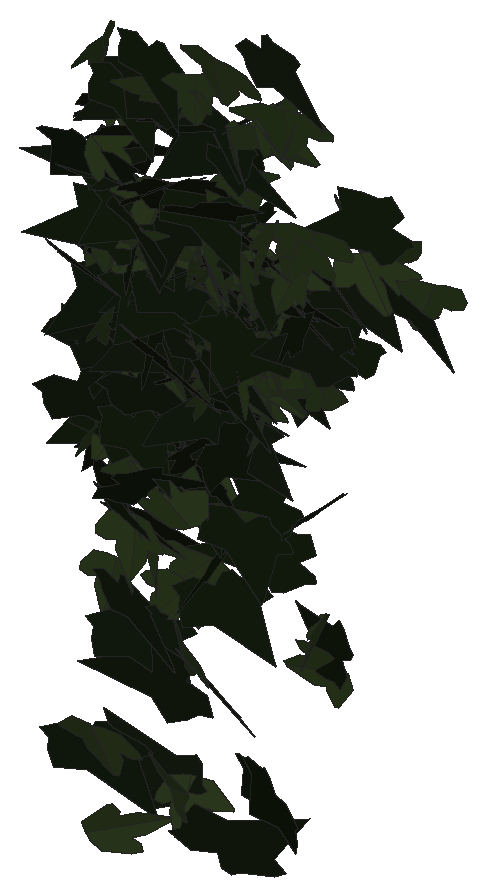
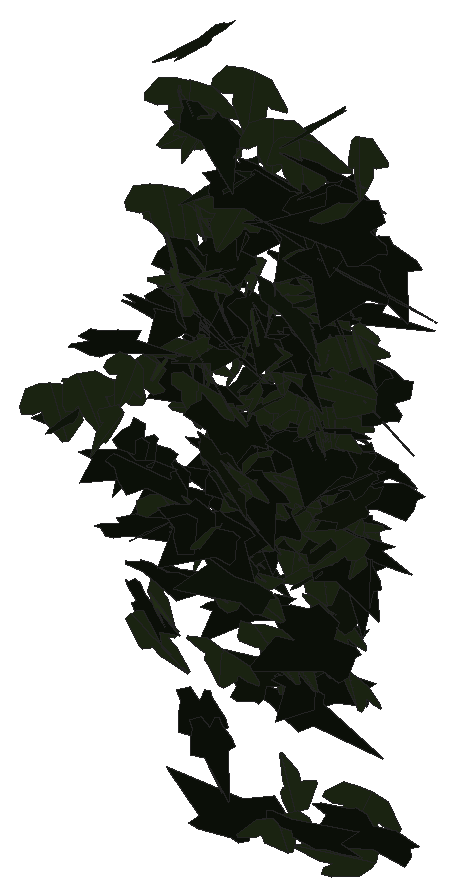
# SketchUp Ruby script. Lengths in millimetres.
U = 1.mm
M = Sketchup.active_model
def pt(a) = Geom::Point3d.new(a.map { |v| v * U })
def face(e, loops, mat)
  f = e.add_face(loops[0].map { |a| pt(a) })
  loops[1..].each { |l| e.add_face(l.map { |a| pt(a) }).erase! }
  f.material = f.back_material = mat if mat
  f
end
# faces: each face lists its corners as indices into pts; further lists are holes
def faces(e, pts, list, mat = nil) = list.each { |f| face(e, (f[0].is_a?(Array) ? f : [f]).map { |l| l.map { |i| pts[i] } }, mat) }
# xy, xz, yz: faces in a plane at the given z, y or x. An outline is a flat list of corners, or four numbers for a rectangle; further outlines are holes
def ring(l) = l.size == 4 ? [[l[0], l[1]], [l[2], l[1]], [l[2], l[3]], [l[0], l[3]]] : l.each_slice(2).to_a
def flat(e, list, mat, &to3) = list.each { |f| face(e, (f[0].is_a?(Array) ? f : [f]).map { |l| ring(l).map { |u, v| to3.(u, v) } }, mat) }
def xy(e, z, list, mat = nil) = flat(e, list, mat) { |x, y| [x, y, z] }
def xz(e, y, list, mat = nil) = flat(e, list, mat) { |x, z| [x, y, z] }
def yz(e, x, list, mat = nil) = flat(e, list, mat) { |y, z| [x, y, z] }
def lines(e, pts, list) = list.each { |a, b| e.add_line(pt(pts[a]), pt(pts[b])) }
# prism: a flat outline (further loops are holes) pulled along v
def prism(e, loops, v, mat = nil)
  f = face(e, loops, mat); d = Geom::Vector3d.new(v.map { |x| x * U })
  f.pushpull(f.normal.samedirection?(d) ? d.length : -d.length)
end
def box(e, o, s, mat = nil) = prism(e, [[o, [o[0] + s[0], o[1], o[2]], [o[0] + s[0], o[1] + s[1], o[2]], [o[0], o[1] + s[1], o[2]]]], [0, 0, s[2]], mat)
def at(x, y, z, deg = 0) = Geom::Transformation.translation(pt([x, y, z])) * Geom::Transformation.rotation(ORIGIN, Z_AXIS, deg.degrees)
def axes(o, x, y, z) = Geom::Transformation.new([*x, 0, *y, 0, *z, 0, *pt(o).to_a, 1])
def part(name) = M.definitions.add(name)
# library, detail: a bought-in or finely detailed component or shape, given as its bounding box
def library(name, o, s) = part(name).tap { |d| box(d.entities, o, s) }
def detail(e, o, s) = box(e.add_group.entities, o, s)
def put(e, d, t, mat = nil) = e.add_instance(d, t).tap { |i| i.material = mat if mat }
def group(e, t, mat = nil) = e.add_group.tap { |g| g.transformation = t; g.material = mat if mat }.entities
root = M.entities
M.materials.add("efeu1").color = [18, 25, 13]
M.materials.add("efeu2").color = [43, 57, 29]
c1 = part("ivyleaf_9")
p = [[39.1,54.8,31.7],[34.5,51.8,30.2],[-5.3,25.2,17.3],[-17.9,28.3,20.9],[-21.6,21.7,17],[-20.2,4.3,5.3],
  [-22.9,-0.3,2.5],[-17.1,-4,-0.6],[-2,-2.1,-1.2],[-0.7,-15.4,-10.1],[16.6,-22.3,-16.7],[21.1,-15.1,-12.5],
  [32.7,-10.7,-11],[46.1,-1.8,-6.6],[30.8,11.2,3.8]]
faces(c1.entities,p,[[0,1,2,3,4,5,6,7,8,9,10,11,12,13,14]],"efeu1")
c2 = part("ivyleaf_10")
p = [[0,12.8,-0.8],[-1.5,51.3,-10.9],[-4.9,51,-11.6],[-13.6,26.5,-7.3],[-13.2,15.9,-4.6],[-21.1,19.3,-7.2],
  [-29.5,16.3,-8.3],[-29.2,8.3,-6.2],[-19.7,-9.8,0.5],[-7.6,-13,4],[1,-12.2,5.8],[-0.4,51.1,-11.1],
  [-1.5,51.1,-10.9],[1,-12.4,5.9],[16.9,-12.4,3.5],[35.1,9.1,-5.1],[35,12.9,-6.1],[20.5,16.4,-4.9],
  [15.8,15,-3.8],[15.3,27.6,-7.1],[12.8,31.3,-7.8]]
faces(c2.entities,p,[[0,1,2,3,4,5,6,7,8,9,10],[11,12,0,13,14,15,16,17,18,19,20]],"efeu2")
put(root,c1,axes([4036.5,844.8,2425.9],[0.72675,0.87653,-0.35288],[-0.34842,-0.30477,-0.95512],[-1.76426,0.42126,0.04326]))
put(root,c1,axes([3981.4,834.6,2057.9],[0.12085,0.58103,-0.82301],[0.24723,0.81303,0.58402],[1.90136,-0.14265,-0.02363]))
put(root,c1,axes([4072.6,839.5,2412.5],[1.22858,0.73783,0.06675],[0.08455,0.04982,-0.98036],[-1.40743,0.64706,-0.00063]))
put(root,c2,axes([3948.9,851.6,2241.1],[0.13677,-0.95686,-0.27886],[0.1005,0.28284,-0.95693],[1.89418,0.05408,0.0709]))
put(root,c2,axes([4040.7,853.5,2035.3],[1.2774,0.03768,0.70919],[-1.3479,-0.03699,0.67224],[0.10044,-0.97574,0.0019]))
put(root,c1,axes([3988.9,868.4,2556.6],[0.22412,-1.0127,0.1095],[0.0018,-0.11012,-1.01945],[1.9386,0.11718,-0.01171]))
put(root,c1,axes([4171.5,844.4,1752],[0.80253,-0.05463,-1.11509],[-2.08064,0.22152,-0.42426],[0.43089,1.1714,0.02823]))
put(root,c1,axes([3976.8,874.3,2352.2],[-0.13475,-0.82447,0.54371],[0.33461,-0.54692,-0.80645],[1.8496,0.03888,0.1855]))
put(root,c2,axes([4017.8,867.2,1695],[-0.99724,0.2867,0.78315],[1.16495,-0.49599,0.59111],[1.07806,0.80118,0.08569]))
put(root,c2,axes([3952.3,841.1,1634.5],[-0.24236,-0.32235,0.95032],[0.62463,0.89188,0.3465],[-1.80484,0.35196,-0.0077]))
put(root,c2,axes([4148.8,866.1,2399.1],[0.28682,-0.92178,0.36124],[0.32407,-0.33582,-0.92796],[1.85616,0.20107,0.1062]))
put(root,c1,axes([3973.5,858.2,2216],[1.68374,-0.52294,0.2093],[0.32287,-0.12423,-1.02749],[1.02224,0.90058,-0.0202]))
put(root,c1,axes([3957.6,871.3,2336.3],[-1.4048,-0.23105,0.65374],[-1.13334,-0.27786,-0.77057],[0.67595,-0.94604,0.06666]))
put(root,c1,axes([3986.4,873.6,2369.2],[-1.49607,-0.49452,0.32912],[-0.39656,-0.28168,-0.92089],[1.05873,-0.8043,0.12015]))
put(root,c1,axes([4084.2,865.5,1993.1],[-0.9583,0.53268,-0.69719],[0.87608,-0.52394,-0.73276],[-1.42157,-0.68197,0.0184]))
put(root,c1,axes([4062.3,865.2,2408.9],[-0.24638,-0.92337,-0.34098],[0.35125,0.31505,-0.92321],[1.84012,-0.18377,0.13057]))
put(root,c1,axes([4003,868.6,2367.5],[-1.35838,-0.18844,-0.70116],[1.35902,-0.00441,-0.7257],[0.24985,-1.00051,0.13525]))
put(root,c2,axes([3996.7,857,2343.4],[-1.81782,-0.12192,-0.11588],[0.22257,-0.00111,-0.96276],[0.23009,-0.96214,0.0158]))
put(root,c1,axes([4145,862.2,2611.8],[0.80477,-0.89334,-0.27629],[-0.06936,0.28725,-0.98456],[1.77832,0.41548,0.08663]))
put(root,c1,axes([3923.6,855.3,2422.1],[0.91515,0.32099,-0.82246],[-1.40893,-0.36372,-0.57477],[-0.91558,0.88054,0.0624]))
put(root,c2,axes([4104.6,868.2,2345.1],[-0.89759,0.60758,-0.59573],[0.43993,-0.56402,-0.75824],[-1.55855,-0.50912,0.12906]))
put(root,c1,axes([3949.2,870.4,1908.8],[0.8109,-0.98165,0.06298],[0.05458,-0.05621,-1.07013],[1.87133,0.42702,0.00392]))
put(root,c1,axes([4054.5,877,1834.2],[0.44139,-0.68251,0.66954],[0.58544,-0.59906,-0.71722],[1.72288,0.37842,0.07218]))
put(root,c1,axes([3968,869.8,2112],[0.0486,-0.93186,-0.28019],[0.05446,0.28089,-0.93156],[1.85115,0.0162,0.03476]))
put(root,c2,axes([4049.6,854.3,1877],[-1.15947,0.60562,0.52098],[-0.74389,0.34544,-0.85863],[-1.32601,-0.72335,0.02614]))
put(root,c2,axes([3937.3,853.8,2431.4],[0.17379,0.88481,0.46957],[0.02273,0.47053,-0.88892],[-1.90628,0.08628,0.03221]))
put(root,c2,axes([3987.7,870.1,2336.3],[1.55558,0.37506,-0.39642],[-0.705,-0.14296,-0.89901],[-0.7627,0.89709,0.02247]))
put(root,c2,axes([3997.5,876.6,2389.3],[-1.02684,-0.76061,0.36563],[0.18223,-0.48633,-0.87041],[1.59579,-0.43389,0.33467]))
put(root,c2,axes([4086.9,861.5,2574.8],[-1.82751,0.28164,0.17703],[-0.30686,0.07902,-1.00023],[-0.55379,-0.97321,-0.02998]))
put(root,c1,axes([3951,875.9,2504.7],[0.02335,-1.00353,-0.14543],[-0.02007,0.14531,-1.00357],[1.92976,0.01365,-0.00868]))
put(root,c1,axes([3993.4,875.7,2510.8],[-1.89727,0.00409,0.06429],[-0.12256,-0.08931,-0.99288],[0.00321,-0.99495,0.08939]))
put(root,c2,axes([4080.3,857.8,2339.1],[-0.8045,0.87477,0.34227],[-0.29796,0.30447,-0.97151],[-1.76276,-0.4507,0.00801]))
put(root,c1,axes([4108.7,877.5,2034.4],[-0.35683,-0.97188,-0.17149],[0.05849,0.16873,-0.9898],[1.87735,-0.18998,-0.00176]))
put(root,c2,axes([4014.2,867.1,2517.6],[-1.74926,-0.38725,0.12108],[-0.20599,-0.05495,-0.99733],[0.74422,-0.92543,0.00855]))
put(root,c1,axes([4003.2,848.1,2402.1],[0.90694,0.74019,0.50477],[0.36079,0.47548,-0.87621],[-1.66651,0.50576,0.08501]))
put(root,c1,axes([4083.3,876.8,2479.3],[-1.91669,0.01537,-0.0447],[0.08402,-0.03504,-1.00662],[-0.03216,-1.00747,0.03433]))
put(root,c2,axes([3921.8,866.1,1728.4],[-1.74339,0.14415,-0.09368],[0.17706,-0.01147,-0.9273],[-0.27515,-0.92074,-0.00312]))
put(root,c1,axes([4030.1,869.3,1827.5],[-0.39088,-0.09178,-1.05774],[-1.864,-0.39954,0.22484],[-0.78008,1.00068,-0.00725]))
put(root,c2,axes([4099.3,868.8,2490.2],[-0.42358,0.96964,-0.12982],[0.01703,-0.13111,-0.99464],[-1.8618,-0.2218,0.02044]))
put(root,c1,axes([3993.4,885.9,2261.5],[-1.25781,-0.65263,0.2339],[-0.19447,-0.22792,-0.92468],[1.30504,-0.66298,0.08765]))
put(root,c2,axes([4167.5,869.9,2538.4],[-1.82818,-0.33509,0.03934],[-0.06118,-0.02726,-1.01724],[0.6392,-0.961,0.01514]))
put(root,c1,axes([3950.7,882.1,2335.9],[-0.8004,0.14549,-0.8766],[1.53067,-0.35005,-0.44395],[-0.71909,-0.90706,0.03072]))
put(root,c1,axes([4114.5,882.3,2254.5],[-1.54837,-0.48363,-0.08834],[0.13424,0.05422,-0.9464],[0.92599,-0.81655,-0.01052]))
put(root,c2,axes([3925.7,866,2549.1],[-0.15213,-0.92921,-0.42172],[0.09813,0.41879,-0.93253],[1.9396,-0.09407,0.0141]))
put(root,c1,axes([3901.8,863.9,2134.3],[-0.27778,-0.31953,-0.94406],[0.60626,0.88913,-0.35019],[1.79738,-0.34929,-0.02778]))
put(root,c1,axes([4090.7,857.6,2131.6],[0.27318,-0.32176,-1.03633],[-0.94992,0.90864,-0.35124],[1.83379,0.51861,-0.02757]))
put(root,c1,axes([3934.2,876.8,2253.8],[-1.83322,0.50519,-0.32722],[0.55131,-0.15219,-1.08767],[-1.00417,-1.00584,0.00022]))
put(root,c2,axes([4043.7,874.4,2535.6],[-1.16482,-0.79543,-0.0282],[0.24436,-0.06355,-0.99376],[1.49497,-0.60937,0.14046]))
put(root,c2,axes([4095,881.4,2216.6],[-0.23503,0.80902,-0.56806],[0.20607,-0.55796,-0.81817],[-1.87006,-0.16316,-0.01876]))
put(root,c2,axes([3973.9,880.1,2058.1],[-0.62642,-0.89291,0.23218],[0.03117,-0.25213,-0.94641],[1.75562,-0.31412,0.09965]))
put(root,c1,axes([4006,883.1,2209.5],[-1.75507,-0.08295,0.1596],[-0.29419,-0.06083,-0.92474],[0.17505,-0.9339,0.04606]))
put(root,c1,axes([4066.4,881.7,2195.6],[0.77653,-0.8839,0.00025],[0.08161,0.01952,-0.97238],[1.68025,0.40755,0.04711]))
put(root,c1,axes([3979.2,886.1,2227.6],[-0.84835,0.22398,-0.81419],[1.37798,-0.37242,-0.49884],[-0.82707,-0.85024,0.00402]))
put(root,c1,axes([4017.7,884.1,2284.7],[-1.81939,-0.01075,0.11059],[-0.21054,0.00256,-0.95602],[0.01976,-0.96234,-0.00377]))
put(root,c1,axes([4084.4,871.8,2469.1],[1.20675,-0.63454,-0.47128],[-0.29913,0.49089,-0.87241],[1.47426,0.619,0.20875]))
put(root,c1,axes([3964.2,864.1,2460.8],[0.68234,0.92403,-0.00446],[0.00468,-0.00573,-0.99114],[-1.75863,0.3585,-0.00437]))
put(root,c1,axes([4138.5,867.4,1741.4],[0.62534,0.05784,-0.91194],[-1.71584,0.17845,-0.31351],[0.28341,0.95276,0.11408]))
put(root,c2,axes([4133.8,870.9,2512.3],[-1.23518,-0.33875,-0.68806],[1.15817,0.32111,-0.73209],[0.88832,-0.88967,-0.00225]))
put(root,c2,axes([4162.9,881.4,2532.6],[0.91494,-0.88459,-0.03625],[0.15026,0.08391,-1.00083],[1.67826,0.47474,0.10937]))
put(root,c1,axes([4080.3,872,1642.8],[-0.56648,0.04063,1.04046],[1.97394,-0.08423,0.29999],[0.17544,1.07892,-0.01576]))
put(root,c2,axes([4193.8,880.2,2401.4],[-1.69724,-0.36298,0.18579],[-0.29848,-0.10711,-0.96202],[0.71637,-0.90461,0.03936]))
put(root,c2,axes([4162.9,883.7,2347.2],[1.35907,-0.69206,-0.00415],[-0.00694,0.0022,-0.99443],[1.31714,0.71411,-0.00095]))
put(root,c1,axes([3964.4,876.5,1869.5],[-0.34243,-0.67367,-0.8148],[0.32671,0.79693,-0.6968],[1.98541,-0.24733,-0.02587]))
put(root,c1,axes([3900.6,881,1709.7],[-0.5795,-0.36779,-0.9293],[1.3907,0.58084,-0.46931],[1.29769,-0.78672,0.08795]))
put(root,c2,axes([4178.7,878.2,2387.6],[-1.73159,0.25476,0.26269],[-0.5495,-0.06724,-0.93478],[-0.42789,-0.9446,0.13739]))
put(root,c1,axes([4051.9,887.4,2148.2],[-1.76431,0.10042,-0.11636],[0.20916,-0.06422,-0.93102],[-0.20449,-0.93209,0.05161]))
put(root,c1,axes([3868,887.1,2260.4],[1.16795,-0.6177,0.43655],[0.72777,-0.23167,-0.86535],[1.24205,0.71659,0.09654]))
put(root,c1,axes([3942.9,881.4,2400.3],[-1.33995,0.61197,0.32245],[-0.87584,-0.07089,-0.87026],[-0.98286,-0.77112,0.3359]))
put(root,c1,axes([4068.6,879.5,2219],[1.08219,-0.66423,-0.43717],[-0.39809,0.39358,-0.87005],[1.46011,0.59962,0.08681]))
put(root,c1,axes([4017.9,894,2054.9],[0.31191,-1.02315,0.03667],[0.0043,-0.03678,-1.03618],[1.9485,0.16386,-0.00359]))
put(root,c1,axes([3972.2,874.7,2159.5],[-0.10814,-0.24632,-0.93817],[0.6531,0.87389,-0.25023],[1.72665,-0.34598,0.03589]))
put(root,c1,axes([4067.7,885.8,2468.7],[0.55157,0.43572,-0.848],[-0.91453,-0.69875,-0.52326],[-1.56718,0.56111,0.00689]))
put(root,c1,axes([4088.7,882.3,2371.8],[1.71802,-0.4291,-0.02418],[-0.04872,0.00248,-0.99946],[0.81651,0.90302,-0.00875]))
put(root,c2,axes([4055.2,888.4,2173.8],[0.10237,-0.96605,0.06532],[0.04247,-0.06416,-0.96736],[1.84229,0.05516,0.01867]))
put(root,c2,axes([3911.1,886.7,2323],[0.36275,-0.96153,-0.07796],[-0.09044,0.07002,-0.97969],[1.83377,0.19366,-0.03289]))
put(root,c1,axes([4055,886.3,2110.2],[-0.33378,0.8742,-0.61157],[0.26974,-0.5952,-0.89144],[-2.0125,-0.22476,-0.01805]))
put(root,c1,axes([3901.8,893.2,2187],[-1.38296,-0.26809,-0.54356],[1.00173,0.14162,-0.77348],[0.57191,-0.89634,0.04037]))
put(root,c1,axes([3939.7,896.1,2091.9],[-0.95422,-0.7549,-0.20222],[0.26366,0.1506,-0.90569],[1.46382,-0.51922,0.03131]))
put(root,c2,axes([3966.5,902.5,1930.9],[-0.50313,0.12261,0.94128],[1.06487,-0.76918,0.25733],[1.45937,0.60353,0.13674]))
put(root,c2,axes([3971.2,893,2190.2],[1.10377,-0.26114,0.70926],[1.32077,-0.17015,-0.63011],[0.56981,0.90024,0.08665]))
put(root,c2,axes([3934.1,892,2088.8],[1.44935,0.42114,-0.32079],[-0.55351,-0.1368,-0.87],[-0.84191,0.81494,0.01974]))
put(root,c1,axes([4026.8,895.6,2034.2],[1.02258,-0.80259,0.13286],[0.10937,-0.12138,-0.96563],[1.5444,0.54,-0.01958]))
put(root,c1,axes([4063.5,886.3,1939.3],[-0.03163,-0.77044,-0.77265],[0.06289,0.77203,-0.77053],[2.07568,-0.03513,0.01157]))
put(root,c2,axes([3942.2,895.9,1965.8],[1.66519,-0.39676,0.27622],[0.46275,-0.13251,-0.9605],[0.79525,0.90789,-0.01948]))
put(root,c2,axes([4136,881.6,2515.8],[0.06084,0.96101,0.29051],[-0.03058,0.29111,-0.96123],[-1.9105,0.02594,0.02464]))
put(root,c2,axes([3942.4,890.7,2225.5],[0.44029,-0.92137,-0.0694],[0.4475,0.12789,-0.91412],[1.70064,0.20489,0.25851]))
put(root,c1,axes([4212.9,894.6,2264.9],[-1.54091,0.2299,0.44537],[-0.88155,-0.01997,-0.83173],[-0.3644,-0.92384,0.12881]))
put(root,c2,axes([4037.9,881,2331.2],[0.41029,-0.79613,-0.5806],[0.20953,0.61008,-0.79566],[1.86358,0.10668,0.21728]))
put(root,c2,axes([4110.1,891,2338.6],[0.55547,0.91319,-0.1306],[-0.07479,-0.12455,-0.9587],[-1.75408,0.2945,-0.00048]))
put(root,c2,axes([3930.3,895.8,2309.6],[-0.99589,-0.80541,0.20904],[-0.05961,-0.2277,-0.9557],[1.58253,-0.51542,0.09555]))
put(root,c1,axes([4116.4,903.5,2337.4],[-0.50829,-0.92883,-0.00992],[0.01668,0.0078,-0.96644],[1.76776,-0.26714,0.00627]))
put(root,c1,axes([3910.7,880.4,2295.5],[1.69583,0.08996,0.39688],[0.72595,0.14832,-0.88998],[-0.26991,0.96409,0.09988]))
put(root,c2,axes([3934.7,884.6,2478.1],[0.28431,0.96069,0.23258],[-0.00258,0.23542,-0.97155],[-1.8812,0.14487,0.03648]))
put(root,c1,axes([3965.8,898.1,2073.7],[0.9445,-0.78109,0.08696],[0.07213,-0.07894,-0.92535],[1.49402,0.49761,-0.0103]))
put(root,c2,axes([4033.3,891.1,2206.9],[-1.7513,-0.18524,0.08099],[-0.13184,-0.06571,-0.93728],[0.36148,-0.9214,0.05056]))
put(root,c1,axes([4012.1,897.2,2225],[0.6419,-0.90199,-0.17381],[0.03526,0.1918,-0.95938],[1.74789,0.32738,0.08318]))
put(root,c1,axes([4010.6,904.7,2238.7],[-0.84304,-0.84214,-0.07989],[0.03416,0.08081,-0.95128],[1.60959,-0.44279,-0.02166]))
put(root,c1,axes([4036.3,906.6,2288.9],[-0.92656,-0.8272,-0.06062],[0.10965,0.03639,-0.95933],[1.57473,-0.48925,0.03113]))
put(root,c1,axes([4125.3,882.8,2524.7],[-0.11163,0.99871,0.08408],[0.00724,0.08445,-1.00039],[-1.90746,-0.05813,-0.00872]))
put(root,c2,axes([4017.1,899.9,1682.2],[0.98114,0.7927,-0.31086],[-0.29436,-0.27017,-0.94544],[-1.59356,0.53796,-0.01675]))
put(root,c2,axes([3964.2,885.9,2298.7],[-0.96183,0.74211,0.40736],[-0.48029,0.32079,-0.89749],[-1.53792,-0.5643,0.02552]))
put(root,c2,axes([3905.5,883.7,2078.7],[-0.16369,-0.67643,-0.77219],[0.20815,0.76444,-0.68183],[1.94264,-0.13891,0.00799]))
put(root,c2,axes([4083.5,883.9,2427.7],[0.888,0.71175,0.52826],[-0.12401,0.6229,-0.78172],[-1.68236,0.32977,0.33645]))
put(root,c2,axes([3908.7,902.9,1904],[1.41689,-0.49476,0.19832],[0.31151,-0.11202,-0.89388],[0.96544,0.76225,-0.00264]))
put(root,c1,axes([4008,897.7,2092],[0.64575,-0.52183,0.748],[-0.84896,0.60117,0.62174],[-1.51402,-0.55966,-0.0296]))
put(root,c1,axes([4064.3,898,2126.2],[-0.23297,-0.57909,-0.75326],[0.99865,0.59196,-0.54035],[1.50751,-0.48163,0.24155]))
put(root,c1,axes([4165,877.2,2266],[0.33378,0.16443,1.06836],[0.17694,1.07602,-0.18087],[-2.04962,0.11967,0.15837]))
put(root,c1,axes([3909.4,879.2,2459.1],[1.05127,0.18946,0.9452],[1.47514,0.56045,-0.5653],[-1.09089,0.94044,0.14646]))
put(root,c1,axes([3911.3,887.6,2035.1],[0.90819,-0.06255,-0.84979],[-1.56133,0.22953,-0.47757],[0.43832,0.94719,0.05961]))
put(root,c2,axes([4012.9,902.5,2278.2],[1.70646,-0.22558,0.30391],[0.56992,-0.05509,-0.92438],[0.44052,0.94512,0.01865]))
put(root,c2,axes([4113.1,903.9,2240.6],[-0.8101,0.68254,-0.49002],[0.32452,-0.46772,-0.79958],[-1.56585,-0.45005,0.0878]))
put(root,c2,axes([4080.4,899.4,2025.7],[-1.48375,-0.48598,0.17593],[-0.27742,-0.09874,-0.91865],[0.94374,-0.79309,0.00656]))
put(root,c2,axes([4004,899.5,1910.8],[1.46163,-0.43627,-0.30648],[-0.50951,0.14923,-0.88325],[0.87753,0.8133,-0.00234]))
put(root,c1,axes([4194,889.9,2074.9],[-0.30941,0.93149,-0.01676],[0.06065,-0.01144,-0.94512],[-1.77207,-0.16303,-0.02942]))
put(root,c2,axes([4121.5,896.9,2321.5],[-1.42235,-0.56666,-0.24156],[0.44469,0.09064,-0.93551],[1.08476,-0.78017,0.06677]))
put(root,c2,axes([4120.2,903.3,2317.8],[-0.63063,-0.90238,0.10754],[0.02286,-0.1188,-0.95989],[1.72942,-0.32748,0.0519]))
put(root,c1,axes([4133.4,887.7,2349.6],[0.60423,0.91527,-0.10994],[-0.204,-0.07884,-0.96586],[-1.74256,0.3266,0.07495]))
put(root,c1,axes([4020.3,885,2335.8],[-0.31767,0.89382,0.39563],[-0.32445,0.36859,-0.90464],[-1.8318,-0.22029,0.09162]))
put(root,c2,axes([4090.5,906.1,2311.5],[0.75961,-0.86014,0.1705],[0.18498,-0.14278,-0.94783],[1.65859,0.40986,0.02762]))
put(root,c1,axes([4038.5,891.4,2071.4],[1.05142,0.01098,-0.77637],[-1.47285,0.08519,-0.54947],[0.12004,0.94905,0.05831]))
put(root,c1,axes([3920,894.6,1988.8],[1.59491,-0.38885,-0.28194],[-0.30376,0.30932,-0.90101],[0.86218,0.8283,0.20411]))
put(root,c2,axes([4031.2,908.6,2049],[0.657,0.71969,-0.48793],[-0.47491,-0.4209,-0.79736],[-1.58523,0.42437,0.03665]))
put(root,c2,axes([4105.9,914.2,2150.4],[-0.34161,0.58583,-0.72328],[-0.25984,-0.74521,-0.56971],[-1.75228,-0.0037,0.22549]))
put(root,c1,axes([4058.6,907.4,2292],[0.76013,-0.2927,0.82257],[1.24837,-0.49641,-0.49513],[1.0967,0.76794,-0.00653]))
put(root,c2,axes([4022.5,895.4,2281.4],[-1.50318,0.38087,0.39228],[-0.68252,0.15937,-0.87679],[-0.78549,-0.86735,0.01115]))
put(root,c1,axes([3994,897.9,1678.3],[-1.82352,-0.20161,-0.2108],[-0.38954,-0.05099,0.97908],[-0.39552,0.97972,0.00758]))
put(root,c2,axes([3988.2,903.1,2197],[0.84466,-0.8263,-0.21183],[-0.21094,0.18091,-0.93787],[1.60971,0.45729,-0.01174]))
put(root,c2,axes([4175.7,912.1,2203.5],[-0.5672,0.71193,0.55488],[0.40388,-0.5127,0.77179],[1.66973,0.36585,0.0018]))
put(root,c2,axes([4146.2,909.8,2326.5],[0.68054,-0.85019,-0.25363],[0.16691,-0.23825,0.92226],[-1.68027,-0.36801,-0.01111]))
put(root,c1,axes([3921.7,914.7,2081.7],[-1.60402,-0.26458,0.25581],[-0.47416,-0.06034,-0.88321],[0.51553,-0.8787,-0.01638]))
put(root,c1,axes([4033.8,886.1,2307.5],[0.51315,0.86857,0.37033],[0.15587,0.36217,-0.90906],[-1.79027,0.28049,0.027]))
put(root,c2,axes([4041.9,903.6,2308.5],[0.21333,-0.94137,-0.19562],[-0.03792,0.19463,-0.94802],[1.8295,0.1138,0.00316]))
put(root,c1,axes([3948.7,911.5,2222.8],[0.90571,-0.82238,0.09023],[0.16083,-0.05523,-0.94907],[1.56632,0.48121,0.04528]))
put(root,c1,axes([3923.4,891.8,2412],[1.2297,0.74725,-0.03278],[-0.0316,-0.02899,-0.98783],[-1.42318,0.6463,-0.0064]))
put(root,c2,axes([4085.2,915.7,2201.1],[0.73227,-0.56527,-0.65372],[0.71315,-0.5357,0.68377],[-1.48214,-0.53704,0.00602]))
put(root,c2,axes([4177.4,911.1,2208.2],[-0.91981,-0.23982,0.78297],[-1.32781,-0.35542,-0.53951],[0.81597,-0.84871,0.00468]))
put(root,c2,axes([4053.1,898.5,2294.7],[-0.60294,0.86538,0.28397],[-0.25335,0.25344,-0.92084],[-1.71479,-0.34172,0.0362]))
put(root,c1,axes([3949.9,920,2209.5],[-0.92818,-0.79464,-0.1327],[0.29023,0.06126,-0.92731],[1.50558,-0.5017,0.09695]))
put(root,c2,axes([4171.6,920.2,1920.4],[0.62632,-0.77667,0.49021],[0.33126,-0.45856,-0.84336],[1.71629,0.37193,-0.01612]))
put(root,c2,axes([4122.7,908.2,2328.3],[1.52801,0.50413,0.0797],[0.10598,0.06115,-0.94776],[-0.96557,0.80449,0.0221]))
put(root,c2,axes([4120.9,903.7,2233],[0.41523,-0.8252,-0.39831],[-0.02618,0.40645,-0.84959],[1.7437,0.20261,0.0821]))
put(root,c2,axes([3935.9,912.4,2225.7],[-1.06757,-0.76683,0.04934],[0.12391,-0.1083,-0.94294],[1.45718,-0.55259,0.11633]))
put(root,c2,axes([4134.7,912.8,2242.4],[-1.80258,-0.05365,0.0742],[-0.10403,-0.28729,-0.90549],[0.1398,-0.90556,0.28288]))
put(root,c1,axes([4007.6,901.3,2293.1],[0.35851,0.06026,-0.95069],[-1.8119,0.04526,-0.18577],[0.0624,0.96811,0.06787]))
put(root,c2,axes([4022.3,920.5,2097.8],[0.67981,-0.1859,0.84769],[1.42861,-0.39386,-0.40267],[0.8289,0.83129,-0.00122]))
put(root,c1,axes([3987.4,890.4,2150],[1.30336,0.62,0.54441],[0.67407,0.4181,-0.92169],[-1.41829,0.76848,0.06224]))
put(root,c1,axes([3916.6,908.8,2059.4],[0.03584,0.78936,-0.47762],[0.01447,-0.47783,-0.78941],[-1.75584,0.01218,-0.01626]))
put(root,c1,axes([3943,904.4,2088.6],[1.73496,-0.15725,-0.03229],[-0.03935,0.06961,-0.92277],[0.30297,0.90951,0.06504]))
put(root,c2,axes([4034.7,904.3,2234.8],[-0.36178,0.90219,0.19635],[-0.15211,0.18364,-0.92115],[-1.75065,-0.2024,0.03946]))
put(root,c1,axes([3885.7,911.1,2181.3],[1.43578,-0.54746,-0.08485],[-0.12535,0.0537,-0.9321],[1.04688,0.75726,0.00476]))
put(root,c2,axes([3899.7,906.9,2266.7],[0.04251,-0.04625,-0.96103],[1.81852,0.11382,0.01673],[0.21478,-0.95453,0.04856]))
put(root,c2,axes([4105.5,904.7,2256.3],[0.46949,0.87462,0.26365],[-0.05154,0.27998,-0.90345],[-1.73781,0.22799,0.09802]))
put(root,c2,axes([3939.5,912.5,2160.5],[1.17254,0.68863,-0.07239],[-0.16847,-0.01777,-0.92243],[-1.30702,0.62007,0.05396]))
put(root,c1,axes([4145.9,906,2293.8],[1.53213,-0.25193,-0.4599],[-0.82682,0.15145,-0.84343],[0.5589,0.91468,0.01298]))
put(root,c1,axes([4119.9,917.7,2047.3],[-1.7355,0.24865,0.00545],[-0.01087,-0.00023,-0.94518],[-0.47322,-0.9119,0.00173]))
put(root,c1,axes([3896.7,925.6,2164.1],[-0.12609,-0.92627,0.03449],[-0.01569,-0.03399,-0.92862],[1.76403,-0.06651,-0.00579]))
put(root,c2,axes([3952.7,914,2226.5],[0.72854,-0.85358,-0.16599],[0.01877,0.18561,-0.93173],[1.65485,0.37368,0.08364]))
put(root,c2,axes([3953.8,912.3,2212],[-1.66026,-0.34319,-0.15132],[0.26991,0.05284,-0.93743],[0.66083,-0.8838,0.00272]))
put(root,c1,axes([4065.6,915.3,2273.1],[1.18709,-0.70236,-0.12914],[0.07569,0.20536,-0.92481],[1.35702,0.60295,0.16455]))
put(root,c2,axes([4021.3,922.6,2143.9],[-0.61083,-0.84965,0.21537],[0.15636,-0.25751,-0.89344],[1.66085,-0.28824,0.16332]))
put(root,c2,axes([4080.5,916.2,2191.7],[0.94986,-0.035,0.80259],[1.51566,0.14587,-0.48885],[-0.20116,0.93379,0.10645]))
put(root,c1,axes([4117.6,906.7,2279.3],[-0.89637,0.58512,0.59344],[-0.65454,0.48444,-0.7506],[-1.44475,-0.58251,-0.02813]))
put(root,c2,axes([3962.2,906.6,2088.4],[-0.61501,0.76023,0.42336],[-0.34716,0.3824,-0.8259],[-1.61931,-0.37072,0.01627]))
put(root,c2,axes([3988.6,911.5,2224.8],[-1.49013,0.47162,0.20492],[-0.31373,0.12339,-0.91381],[-0.927,-0.79987,-0.02014]))
put(root,c1,axes([4004,921.1,2136.2],[0.92997,-0.29121,0.74554],[1.21835,-0.38214,-0.56883],[0.91439,0.80533,-0.00033]))
put(root,c1,axes([3953.1,927.7,2118.4],[0.41389,-0.89595,0.07704],[0.00605,-0.07849,-0.92184],[1.71146,0.21695,-0.01537]))
put(root,c1,axes([4105.4,918.9,2215.8],[-0.54946,-0.15655,-0.88325],[1.44966,0.44727,-0.32825],[0.90167,-0.81451,-0.01049]))
put(root,c2,axes([3947.2,935.6,2076.3],[-0.75235,-0.4169,-0.95431],[-1.1739,-0.72872,0.57385],[-1.59695,0.73208,0.02776]))
put(root,c1,axes([3935.3,926.5,2044.7],[0.66795,-0.85963,-0.00658],[0.05725,0.01938,-0.92785],[1.63509,0.35049,0.03517]))
put(root,c1,axes([4018.5,921.1,2093.4],[0.82888,-0.17995,0.81101],[1.41225,-0.32743,-0.47113],[0.71083,0.86035,-0.00967]))
put(root,c2,axes([4192.8,913.7,1875.7],[0.87749,-0.2348,-0.81317],[-1.20105,0.5217,-0.50845],[1.07344,0.77566,0.09583]))
put(root,c1,axes([4206.9,908.9,1897.9],[-0.93454,0.4243,-0.71417],[-1.4604,0.08611,0.57876],[0.60561,0.8624,0.29358]))
put(root,c2,axes([3972.4,922.8,2066.9],[-1.28981,-0.63529,-0.08735],[0.27085,-0.02508,-0.92175],[1.19003,-0.68285,0.11512]))
put(root,c1,axes([3876.1,927.1,2142.8],[0.9975,-0.76443,-0.03084],[0.11459,0.07848,-0.92208],[1.45153,0.51913,0.09399]))
put(root,c2,axes([4106.3,925.9,2207.8],[1.70423,-0.25647,0.11415],[0.28877,0.12112,-0.91813],[0.44951,0.89454,0.15704]))
put(root,c2,axes([3933.5,926.6,2038.8],[1.01154,0.74323,-0.16148],[-0.25021,-0.10426,-0.91258],[-1.42573,0.54561,0.04558]))
put(root,c1,axes([4125,936.5,1972],[-1.4126,0.15003,0.58821],[-1.15209,-0.11353,-0.73489],[-0.08629,-0.94021,0.1826]))
put(root,c2,axes([3966.4,923.4,2119.6],[-0.35636,-0.03178,-0.91314],[1.69043,0.21231,-0.18952],[0.40789,-0.90764,-0.01236]))
put(root,c2,axes([4010.2,930,1934.2],[1.59076,-0.19406,-0.40644],[-0.69031,0.21792,-0.84995],[0.50818,0.90351,0.11771]))
put(root,c1,axes([3940.4,918.8,2191.9],[0.91511,0.79451,-0.01834],[-0.01693,-0.01606,-0.92868],[-1.51242,0.48091,-0.0007]))
put(root,c1,axes([4065.8,919.7,2187.1],[0.5739,0.88396,0.08357],[0.08583,0.07289,-0.93378],[-1.68767,0.3043,-0.01907]))
put(root,c1,axes([3923.1,926.2,1958.5],[2.11076,-0.06823,0.04669],[0.08907,0.00039,-1.11115],[0.12971,1.11004,0.00326]))
put(root,c1,axes([3918.2,938.3,2095.3],[1.25826,-0.63323,0.0891],[0.11669,-0.0648,-0.91546],[1.21144,0.66395,-0.00436]))
put(root,c2,axes([3988.4,934.8,2133.7],[-1.21396,-0.62642,-0.23611],[0.2822,0.18583,-0.89358],[1.24243,-0.65427,-0.02774]))
put(root,c2,axes([3897.2,929.5,2091.6],[0.75775,0.64141,0.53402],[0.39161,0.49797,-0.75152],[-1.53941,0.4424,0.07168]))
put(root,c1,axes([3999.9,949.5,2109],[1.36179,0.5567,-0.18553],[-0.32806,-0.08027,-0.90563],[-1.06754,0.73482,0.04163]))
put(root,c1,axes([4146.4,1063.8,2316.9],[-1.23947,-0.30049,0.65721],[-1.10798,-0.306,-0.7168],[0.81482,-0.87317,0.02503]))
put(root,c1,axes([3991.6,1046.6,2106.5],[-0.29328,0.45417,0.79811],[-0.86036,0.66689,-0.46678],[-1.52123,-0.46473,0.11013]))
put(root,c2,axes([4121.1,1058.9,2265.4],[1.31135,0.63524,0.26075],[0.32382,0.19993,-0.93667],[-1.26612,0.70906,0.03051]))
put(root,c1,axes([4155.4,1081.8,2234.2],[0.6928,-0.90757,0.07302],[0.06237,-0.06553,-0.97783],[1.73175,0.36544,0.00601]))
put(root,c2,axes([3910.5,1083.3,2217.3],[0.87702,0.56196,-0.60234],[-0.84429,-0.41226,-0.72402],[-1.32107,0.63655,0.06284]))
put(root,c2,axes([3926.1,1085.8,2096.1],[-0.93229,-0.49853,0.65295],[-0.69335,-0.54955,-0.69289],[1.40134,-0.60357,0.09157]))
put(root,c1,axes([4023.8,1089.6,2140.4],[-0.0977,-0.95699,0.09048],[-0.02938,-0.08977,-0.9583],[1.82922,-0.05255,-0.01056]))
put(root,c1,axes([4011.8,1070.1,2181.7],[1.81373,-0.02334,-0.11756],[-0.22322,0.01243,-0.95323],[0.04698,0.96013,0.00949]))
put(root,c1,axes([4072.6,1069,2220.7],[1.30106,-0.26828,-0.63],[-1.06971,0.28861,-0.7328],[0.74435,0.88371,0.04807]))
put(root,c2,axes([4087.5,1073.2,2305.9],[-1.28145,0.66108,0.08074],[-0.11027,0.05623,-0.94359],[-1.2627,-0.6758,0.00047]))
put(root,c2,axes([4025,1083.8,2159.3],[-1.50039,-0.30923,0.46934],[-0.71416,-0.31233,-0.83609],[0.79637,-0.86269,0.13447]))
put(root,c2,axes([3933.3,1083.5,2231.3],[1.68604,-0.31674,0.10492],[0.19931,-0.01868,-0.94065],[0.60294,0.89189,0.01756]))
put(root,c1,axes([3947.7,1074,2209],[-0.93637,0.7917,0.02654],[-0.04327,0.01711,-0.93206],[-1.50699,-0.49241,0.01027]))
put(root,c2,axes([4184.3,1086.6,2244.7],[-1.32875,-0.66785,0.17498],[-0.12981,-0.18092,-0.96265],[1.30752,-0.69665,0.08225]))
put(root,c1,axes([3921.4,1079.3,2228.4],[0.96901,0.1908,-0.77146],[-1.36252,-0.28762,-0.54362],[-0.6566,0.87844,-0.01043]))
put(root,c2,axes([4137.4,1091.8,2275.4],[-0.65145,-0.90405,0.17763],[-0.03898,-0.18198,-0.96566],[1.75306,-0.34,0.04454]))
put(root,c1,axes([4060.7,1092.3,2213.5],[-0.45037,0.61176,-0.66923],[-0.04156,-0.69529,-0.62787],[-1.72515,-0.14296,0.18984]))
put(root,c1,axes([3964.7,1090.2,2159.5],[0.05012,0.74002,-0.55639],[-0.36989,-0.53979,-0.72715],[-1.72282,0.13742,0.13993]))
put(root,c1,axes([3954.9,1076.3,2243.6],[-0.27814,0.84499,0.38648],[-0.12265,0.38107,-0.85753],[-1.76415,-0.15972,-0.00132]))
put(root,c1,axes([4063.3,1112.7,2136.5],[-1.3451,-0.49822,0.42464],[-0.68728,-0.22451,-0.86443],[1.0392,-0.79336,-0.02205]))
put(root,c2,axes([3956.8,1090.6,2153.2],[-0.22194,0.93037,0.21226],[-0.07326,0.20908,-0.93757],[-1.8147,-0.12223,0.01189]))
put(root,c1,axes([4061.9,1099.9,2211.2],[-0.3651,-0.5819,-0.70819],[0.77545,0.59398,-0.59842],[1.56263,-0.43072,0.1315]))
put(root,c1,axes([4002.7,1110.3,2094],[-1.36414,-0.47023,-0.42279],[0.83833,0.08724,-0.84379],[0.86347,-0.82758,0.15128]))
put(root,c1,axes([3952.1,1097,2163.3],[1.74207,0.02089,-0.13093],[-0.24883,-0.00935,-0.91556],[-0.04188,0.92461,-0.0063]))
put(root,c2,axes([4097.7,1088.1,2245.4],[-0.11881,0.46055,0.81864],[-0.40443,0.79225,-0.46191],[-1.74132,-0.21543,0.05143]))
put(root,c2,axes([3922.6,1112.3,2018.6],[1.6941,-0.19193,0.23887],[0.44931,-0.03826,-0.91051],[0.37177,0.92083,0.01195]))
put(root,c1,axes([3903.2,1092.4,2112.2],[1.34635,0.2423,0.59218],[0.64194,0.60895,-0.65209],[-1.03477,0.69303,0.36594]))
